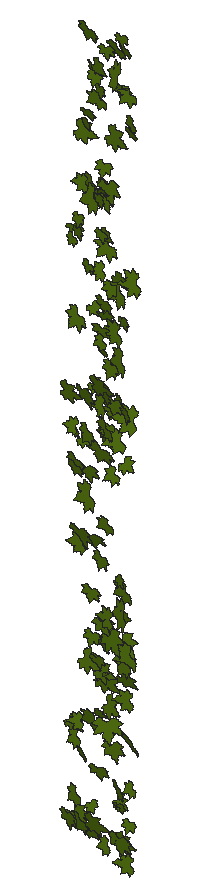
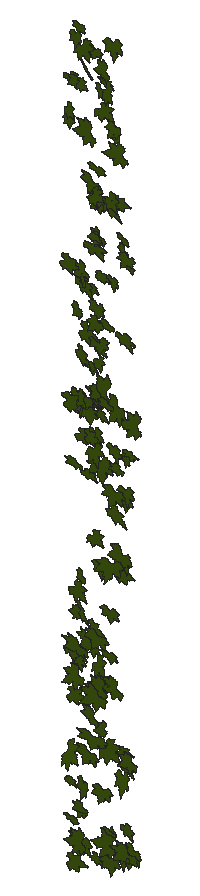
# SketchUp Ruby script. Lengths in inches.
U = 1.inch
M = Sketchup.active_model
def pt(a) = Geom::Point3d.new(a.map { |v| v * U })
def face(e, loops, mat)
  f = e.add_face(loops[0].map { |a| pt(a) })
  loops[1..].each { |l| e.add_face(l.map { |a| pt(a) }).erase! }
  f.material = f.back_material = mat if mat
  f
end
# faces: each face lists its corners as indices into pts; further lists are holes
def faces(e, pts, list, mat = nil) = list.each { |f| face(e, (f[0].is_a?(Array) ? f : [f]).map { |l| l.map { |i| pts[i] } }, mat) }
# xy, xz, yz: faces in a plane at the given z, y or x. An outline is a flat list of corners, or four numbers for a rectangle; further outlines are holes
def ring(l) = l.size == 4 ? [[l[0], l[1]], [l[2], l[1]], [l[2], l[3]], [l[0], l[3]]] : l.each_slice(2).to_a
def flat(e, list, mat, &to3) = list.each { |f| face(e, (f[0].is_a?(Array) ? f : [f]).map { |l| ring(l).map { |u, v| to3.(u, v) } }, mat) }
def xy(e, z, list, mat = nil) = flat(e, list, mat) { |x, y| [x, y, z] }
def xz(e, y, list, mat = nil) = flat(e, list, mat) { |x, z| [x, y, z] }
def yz(e, x, list, mat = nil) = flat(e, list, mat) { |y, z| [x, y, z] }
def lines(e, pts, list) = list.each { |a, b| e.add_line(pt(pts[a]), pt(pts[b])) }
# prism: a flat outline (further loops are holes) pulled along v
def prism(e, loops, v, mat = nil)
  f = face(e, loops, mat); d = Geom::Vector3d.new(v.map { |x| x * U })
  f.pushpull(f.normal.samedirection?(d) ? d.length : -d.length)
end
def box(e, o, s, mat = nil) = prism(e, [[o, [o[0] + s[0], o[1], o[2]], [o[0] + s[0], o[1] + s[1], o[2]], [o[0], o[1] + s[1], o[2]]]], [0, 0, s[2]], mat)
def at(x, y, z, deg = 0) = Geom::Transformation.translation(pt([x, y, z])) * Geom::Transformation.rotation(ORIGIN, Z_AXIS, deg.degrees)
def axes(o, x, y, z) = Geom::Transformation.new([*x, 0, *y, 0, *z, 0, *pt(o).to_a, 1])
def part(name) = M.definitions.add(name)
# library, detail: a bought-in or finely detailed component or shape, given as its bounding box
def library(name, o, s) = part(name).tap { |d| box(d.entities, o, s) }
def detail(e, o, s) = box(e.add_group.entities, o, s)
def put(e, d, t, mat = nil) = e.add_instance(d, t).tap { |i| i.material = mat if mat }
def group(e, t, mat = nil) = e.add_group.tap { |g| g.transformation = t; g.material = mat if mat }.entities
root = M.entities
M.materials.add("[Vegetation Blur 03]").color = [83, 114, 18]
c1 = part("ivy")
xy(c1.entities,0,[[0.782,0,0.786,0,0.787,0.005,0.789,0.009,0.821,0.072,0.875,0.147,1.001,0.272,1.073,0.331,1.137,0.363,1.178,0.379,1.223,0.384,1.272,0.383,1.311,0.374,1.36,0.355,1.399,0.334,1.491,0.285,1.541,0.244,1.583,0.199,1.617,0.15,1.64,0.128,1.662,0.115,1.717,0.105,1.745,0.093,1.784,0.054,1.819,0.057,1.854,0.064,1.882,0.075,1.896,0.074,1.91,0.071,1.937,0.063,1.964,0.053,1.99,0.038,2.016,0.015,2.034,0.002,2.04,0,2.038,0.003,2.036,0.007,2.033,0.038,2.036,0.068,2.045,0.1,2.055,0.116,2.064,0.123,2.077,0.129,2.088,0.129,2.106,0.132,2.118,0.13,2.179,0.132,2.207,0.133,2.225,0.133,2.242,0.138,2.22,0.162,2.207,0.186,2.206,0.213,2.212,0.236,2.228,0.262,2.247,0.274,2.298,0.283,2.355,0.294,2.37,0.296,2.376,0.295,2.377,0.3,2.377,0.303,2.385,0.329,2.411,0.37,2.426,0.392,2.449,0.407,2.511,0.426,2.561,0.444,2.619,0.466,2.589,0.469,2.561,0.476,2.501,0.5,2.449,0.516,2.424,0.523,2.401,0.535,2.377,0.556,2.372,0.568,2.36,0.575,2.268,0.586,2.225,0.592,2.207,0.599,2.194,0.61,2.143,0.65,2.13,0.664,2.122,0.682,2.123,0.7,2.13,0.719,2.148,0.75,2.17,0.781,2.195,0.807,2.221,0.828,2.284,0.874,2.291,0.88,2.288,0.887,2.276,0.9,2.267,0.916,2.265,0.933,2.273,0.967,2.292,1.002,2.313,1.03,2.334,1.054,2.348,1.067,2.358,1.074,2.363,1.076,2.362,1.081,2.35,1.094,2.347,1.11,2.35,1.143,2.359,1.18,2.385,1.254,2.415,1.324,2.448,1.393,2.45,1.4,2.446,1.398,2.44,1.394,2.427,1.383,2.402,1.36,2.376,1.339,2.345,1.324,2.305,1.309,2.282,1.303,2.273,1.306,2.245,1.294,2.212,1.287,2.187,1.291,2.163,1.301,2.142,1.316,2.134,1.327,2.124,1.325,2.09,1.292,2.053,1.259,2.014,1.234,1.973,1.215,1.954,1.21,1.931,1.208,1.909,1.212,1.893,1.22,1.879,1.233,1.872,1.248,1.867,1.281,1.864,1.319,1.821,1.258,1.773,1.197,1.726,1.141,1.698,1.121,1.679,1.116,1.666,1.117,1.647,1.122,1.632,1.129,1.62,1.141,1.617,1.154,1.617,1.219,1.621,1.254,1.623,1.268,1.623,1.281,1.618,1.314,1.606,1.346,1.603,1.375,1.607,1.403,1.603,1.467,1.599,1.499,1.605,1.525,1.614,1.552,1.629,1.577,1.635,1.589,1.629,1.587,1.618,1.582,1.596,1.566,1.581,1.556,1.568,1.552,1.557,1.55,1.545,1.553,1.531,1.562,1.522,1.572,1.504,1.591,1.486,1.611,1.474,1.631,1.457,1.666,1.455,1.684,1.457,1.698,1.452,1.715,1.444,1.728,1.424,1.754,1.419,1.772,1.423,1.786,1.434,1.819,1.444,1.848,1.446,1.855,1.44,1.861,1.43,1.867,1.386,1.904,1.349,1.948,1.326,1.973,1.31,1.995,1.288,2.048,1.284,2.153,1.287,2.254,1.284,2.255,1.282,2.253,1.278,2.247,1.274,2.237,1.266,2.216,1.226,2.125,1.208,2.076,1.184,2.033,1.155,1.984,1.135,1.942,1.111,1.899,1.083,1.861,1.053,1.85,1.059,1.83,1.061,1.809,1.056,1.79,1.049,1.767,1.04,1.749,1.018,1.733,0.994,1.726,0.942,1.734,0.95,1.6875,0.944,1.645,0.932,1.608,0.911,1.585,0.881,1.58,0.854,1.582,0.828,1.588,0.785,1.618,0.773,1.625,0.775,1.614,0.779,1.598,0.796,1.502,0.818,1.402,0.861,1.283,0.882,1.224,0.894,1.174,0.892,1.148,0.886,1.123,0.881,1.107,0.872,1.099,0.849,1.094,0.818,1.092,0.789,1.098,0.762,1.107,0.753,1.113,0.721,1.139,0.698,1.163,0.678,1.194,0.665,1.224,0.628,1.28,0.612,1.312,0.606,1.327,0.606,1.314,0.599,1.282,0.594,1.267,0.581,1.256,0.544,1.245,0.512,1.244,0.473,1.249,0.444,1.256,0.382,1.288,0.339,1.306,0.324,1.316,0.317,1.324,0.309,1.326,0.27,1.314,0.227,1.313,0.185,1.3125,0.152,1.317,0.122,1.328,0.092,1.345,0.073,1.353,0.079,1.338,0.092,1.308,0.117,1.249,0.13,1.215,0.139,1.164,0.147,1.148,0.157,1.136,0.163,1.122,0.174,1.086,0.177,1.067,0.182,1.054,0.186,1.043,0.191,1.038,0.211,1.028,0.237,1.005,0.25,0.974,0.253,0.96,0.25,0.944,0.242,0.914,0.243,0.906,0.249,0.902,0.26,0.894,0.289,0.88,0.307,0.873,0.322,0.862,0.364,0.799,0.403,0.738,0.431,0.709,0.439,0.691,0.441,0.678,0.4375,0.66,0.428,0.645,0.394,0.623,0.303,0.594,0.255,0.581,0.214,0.577,0.179,0.573,0.173,0.568,0.175,0.561,0.167,0.55,0.141,0.523,0.113,0.503,0.077,0.49,0.045,0.486,0.026,0.485,0.019,0.486,0.011,0.483,0,0.471,0.014,0.467,0.044,0.455,0.058,0.447,0.07,0.438,0.097,0.411,0.125,0.394,0.158,0.377,0.174,0.366,0.182,0.359,0.185,0.361,0.242,0.331,0.253,0.316,0.258,0.303,0.262,0.283,0.274,0.278,0.308,0.274,0.341,0.252,0.366,0.226,0.366,0.222,0.37,0.22,0.38,0.221,0.395,0.221,0.425,0.216,0.45,0.207,0.465,0.192,0.473,0.178,0.484,0.15,0.489,0.116,0.483,0.089,0.468,0.058,0.45,0.035,0.435,0.018,0.429,0.011,0.434,0.012,0.438,0.014,0.469,0.019,0.542,0.016,0.581,0.015,0.612,0.027,0.68,0.055,0.696,0.057,0.712,0.052,0.73,0.045,0.741,0.036,0.766,0.014]])
put(root,c1,axes([118.79,173.7,103.93],[0.51714,-0.23527,0.06533],[0.0842,0.02179,-0.43163],[-0.1113,-1.07662,-0.02301]),"[Vegetation Blur 03]")
put(root,c1,axes([119.9,173.7,124.375],[0.04403,-0.12753,-0.27738],[-0.34532,-0.03734,-0.03381],[0.01033,-0.70424,0.05202]),"[Vegetation Blur 03]")
put(root,c1,axes([119.375,173.7,133.94],[0.27643,-0.11245,-0.0959],[-0.1208,-0.01738,-0.22873],[-0.04691,-0.61786,0.02389]),"[Vegetation Blur 03]")
put(root,c1,axes([118.87,173.7,125.11],[0.08822,-0.12322,0.46198],[0.56917,0.00464,-0.0722],[-0.00698,-1.17889,-0.04857]),"[Vegetation Blur 03]")
put(root,c1,axes([119.09,173.7,134.17],[0.33638,0.01493,0.11781],[0.14294,0.07701,-0.27338],[0.02139,-0.74929,-0.02575]),"[Vegetation Blur 03]")
put(root,c1,axes([119.55,173.7,105.4],[0.34978,-0.17504,-0.23097],[-0.28247,0.06704,-0.29293],[-0.08681,-0.92345,0.02252]),"[Vegetation Blur 03]")
put(root,c1,axes([118.95,173.7,108.24],[0.25126,-0.00237,0.3092],[0.37875,0.02524,-0.20497],[0.00958,-0.93516,-0.00632]),"[Vegetation Blur 03]")
put(root,c1,axes([119.3,173.7,122.54],[0.44154,-0.10792,-0.13293],[-0.15664,0.11844,-0.36167],[-0.06888,-0.96117,-0.02964]),"[Vegetation Blur 03]")
put(root,c1,axes([119.32,173.7,122.13],[0.39751,-0.09835,-0.09675],[-0.112,0.11608,-0.32505],[-0.0616,-0.84567,-0.03337]),"[Vegetation Blur 03]")
put(root,c1,axes([120.2,173.7,118.44],[0.06394,-0.03491,-0.38067],[-0.46672,-0.01334,-0.05203],[0.00412,-0.96871,0.01444]),"[Vegetation Blur 03]")
put(root,c1,axes([119.71,173.7,108.375],[0.28202,-0.18926,-0.22565],[-0.28437,-0.00619,-0.23592],[-0.06351,-0.81269,0.05435]),"[Vegetation Blur 03]")
put(root,c1,axes([119.47,173.7,123.98],[0.28723,-0.15203,-0.02555],[-0.02588,0.0511,-0.24162],[-0.07595,-0.59236,-0.01429]),"[Vegetation Blur 03]")
put(root,c1,axes([120.08,173.7,109.22],[0.11929,-0.10597,-0.2818],[-0.34889,-0.06251,-0.09467],[0.01224,-0.74914,0.04776]),"[Vegetation Blur 03]")
put(root,c1,axes([119.54,173.7,130.3],[0.50454,-0.20666,-0.19788],[-0.2502,-0.0525,-0.4163],[-0.0792,-1.15072,0.05453]),"[Vegetation Blur 03]")
put(root,c1,axes([118.85,173.7,103.51],[0.43162,0.02667,0.37239],[0.45622,0.01814,-0.35241],[0.01531,-1.29236,0.00274]),"[Vegetation Blur 03]")
put(root,c1,axes([119.5,173.7,107.9],[0.51252,-0.27009,-0.18144],[-0.18784,0.30748,-0.42542],[-0.17711,-1.10772,-0.07385]),"[Vegetation Blur 03]")
put(root,c1,axes([119.56,173.7,104.04],[0.4822,-0.17189,-0.16775],[-0.19534,0.15084,-0.39833],[-0.10519,-1.06807,-0.02926]),"[Vegetation Blur 03]")
put(root,c1,axes([120.39,173.7,137.16],[0.05825,-0.05857,-0.32384],[-0.39732,-0.0501,-0.04618],[0.02002,-0.82377,0.02584]),"[Vegetation Blur 03]")
put(root,c1,axes([119.58,173.7,135.01],[0.33002,-0.10362,0.05882],[0.06392,-0.11285,-0.27012],[-0.06037,-0.68589,0.03556]),"[Vegetation Blur 03]")
put(root,c1,axes([119.53,173.7,134.21],[0.29872,-0.15455,0.15212],[0.18312,-0.07365,-0.25129],[-0.08276,-0.72081,-0.00694]),"[Vegetation Blur 03]")
put(root,c1,axes([119.71,173.7,123.02],[0.11399,0.08931,0.26369],[0.32563,0.00233,-0.09389],[0.01551,-0.70503,0.03309]),"[Vegetation Blur 03]")
put(root,c1,axes([119.25,173.7,118.8],[0.63866,-0.23189,0.12864],[0.16822,0.10928,-0.52532],[-0.09614,-1.34925,-0.06466]),"[Vegetation Blur 03]")
put(root,c1,axes([120.54,173.7,109.51],[0.24902,0.09318,-0.40988],[-0.50306,0.12516,-0.1991],[-0.03467,-1.14673,-0.05504]),"[Vegetation Blur 03]")
put(root,c1,axes([119.55,173.7,138.76],[0.09049,0.02962,0.47011],[0.57571,0.04471,-0.07426],[0.0237,-1.19903,0.00884]),"[Vegetation Blur 03]")
put(root,c1,axes([120.66,173.7,142.97],[0.14161,0.02749,-0.37414],[-0.43235,0.33737,-0.1051],[-0.153,-0.92792,-0.0493]),"[Vegetation Blur 03]")
put(root,c1,axes([120.43,173.7,121.4375],[0.39569,-0.25539,-0.40505],[-0.50198,0.05522,-0.33211],[-0.09868,-1.305,0.06522]),"[Vegetation Blur 03]")
put(root,c1,axes([119.92,173.7,145.125],[0.51011,-0.11701,-0.13612],[-0.15838,0.15628,-0.41647],[-0.07724,-1.09327,-0.04497]),"[Vegetation Blur 03]")
put(root,c1,axes([120.43,173.7,137.34],[0.31562,-0.0779,-0.30416],[-0.3657,0.1532,-0.25894],[-0.08116,-0.99323,-0.01608]),"[Vegetation Blur 03]")
put(root,c1,axes([120.03,173.7,103.54],[0.43132,0.00683,-0.12215],[-0.14822,0.15148,-0.34728],[-0.02104,-0.9272,-0.05763]),"[Vegetation Blur 03]")
put(root,c1,axes([119.72,173.7,118.54],[0.54712,0.06533,0.00829],[0.00324,0.23778,-0.43729],[0.03318,-1.10066,-0.09398]),"[Vegetation Blur 03]")
put(root,c1,axes([119.68,173.7,122.03],[0.51598,-0.04836,0.08245],[0.10256,0.07999,-0.4201],[-0.01553,-1.07898,-0.03484]),"[Vegetation Blur 03]")
put(root,c1,axes([120.11,173.7,124.36],[0.44792,-0.20906,-0.13241],[-0.16237,0.03502,-0.37455],[-0.10139,-0.9797,0.01487]),"[Vegetation Blur 03]")
put(root,c1,axes([119.91,173.7,140.5],[0.35213,-0.1038,0.09821],[0.12718,0.11373,-0.28482],[-0.02917,-0.75727,-0.05624]),"[Vegetation Blur 03]")
put(root,c1,axes([120.21,173.7,132.87],[0.35103,-0.1488,-0.07514],[-0.0909,0.03087,-0.29249],[-0.07377,-0.74614,0.00288]),"[Vegetation Blur 03]")
put(root,c1,axes([120.04,173.7,139.92],[0.22551,-0.17157,0.19026],[0.23404,-0.06401,-0.19384],[-0.08079,-0.66437,-0.03046]),"[Vegetation Blur 03]")
put(root,c1,axes([120.7,173.7,136.93],[0.36429,-0.26691,-0.39719],[-0.49048,0.09297,-0.30946],[-0.1145,-1.24751,0.06192]),"[Vegetation Blur 03]")
put(root,c1,axes([119.75,173.7,111.54],[0.19537,0.05525,0.44525],[0.54604,-0.05051,-0.1586],[-0.01409,-1.19141,0.02737]),"[Vegetation Blur 03]")
put(root,c1,axes([119.64,173.7,126.11],[0.57292,-0.29787,0.17247],[0.22282,0.05394,-0.47834],[-0.12636,-1.25544,-0.06147]),"[Vegetation Blur 03]")
put(root,c1,axes([120.13,173.7,115.97],[0.45876,-0.06676,-0.02085],[-0.02631,-0.02088,-0.37522],[-0.03182,-0.94526,0.00976]),"[Vegetation Blur 03]")
put(root,c1,axes([120.23,173.7,104.47],[0.21181,0.06558,0.16158],[0.19963,-0.12494,-0.16633],[-0.01894,-0.58339,0.05378]),"[Vegetation Blur 03]")
put(root,c1,axes([120.875,173.7,141.78],[0.26725,0.04128,-0.32232],[-0.39537,0.00799,-0.21819],[0.00802,-0.98126,-0.01534]),"[Vegetation Blur 03]")
put(root,c1,axes([120.28,173.7,113.7],[0.40879,-0.06868,-0.00639],[-0.01176,-0.09983,-0.33231],[-0.0322,-0.83542,0.04024]),"[Vegetation Blur 03]")
put(root,c1,axes([120.27,173.7,130.23],[0.21448,0.07418,0.20841],[0.25788,-0.06923,-0.1729],[-0.00284,-0.68276,0.04017]),"[Vegetation Blur 03]")
put(root,c1,axes([121.09,173.7,113.58],[0.21131,0.04206,-0.34485],[-0.41038,0.25638,-0.16258],[-0.10272,-0.93777,-0.05992]),"[Vegetation Blur 03]")
put(root,c1,axes([120.33,173.7,126.15],[0.18344,0.08958,0.24161],[0.29922,-0.05038,-0.14838],[0.0019,-0.7149,0.04073]),"[Vegetation Blur 03]")
put(root,c1,axes([120.5,173.7,142.72],[0.38042,-0.08348,0.02066],[0.01844,-0.12918,-0.30833],[-0.04412,-0.77385,0.04924]),"[Vegetation Blur 03]")
put(root,c1,axes([120.41,173.7,106.68],[0.44484,-0.01751,0.04002],[0.04967,0.10203,-0.36079],[-0.00297,-0.91526,-0.04099]),"[Vegetation Blur 03]")
put(root,c1,axes([120.47,173.7,112.36],[0.36338,-0.06137,0.0857],[0.10665,0.03955,-0.29676],[-0.02326,-0.77736,-0.02186]),"[Vegetation Blur 03]")
put(root,c1,axes([120.52,173.7,123.66],[0.62172,-0.07982,-0.18766],[-0.22411,0.16779,-0.50577],[-0.06444,-1.35373,-0.05162]),"[Vegetation Blur 03]")
put(root,c1,axes([121.01,173.7,128.71],[0.25042,-0.03463,-0.18206],[-0.21423,0.16131,-0.2011],[-0.06442,-0.671,-0.03895]),"[Vegetation Blur 03]")
put(root,c1,axes([121.46,173.7,137.26],[0.07231,0.11382,-0.30015],[-0.37128,0.06711,-0.05557],[-0.02172,-0.76837,-0.04931]),"[Vegetation Blur 03]")
put(root,c1,axes([121.36,173.7,133.02],[0.14335,-0.13764,-0.29117],[-0.36286,-0.03379,-0.11648],[-0.00945,-0.79049,0.05568]),"[Vegetation Blur 03]")
put(root,c1,axes([121.33,173.7,126.09],[0.18991,-0.19032,-0.31472],[-0.38839,0.08836,-0.16451],[-0.08006,-0.88012,0.05154]),"[Vegetation Blur 03]")
put(root,c1,axes([120.33,173.7,103.26],[0.11966,-0.19885,0.48664],[0.60405,0.04067,-0.09632],[0.00062,-1.25082,-0.0805]),"[Vegetation Blur 03]")
put(root,c1,axes([120.69,173.7,129.65],[0.43667,-0.00599,-0.05285],[-0.0643,0.07555,-0.35518],[-0.00825,-0.90526,-0.02929]),"[Vegetation Blur 03]")
put(root,c1,axes([121.19,173.7,129.25],[0.22039,-0.10268,-0.20891],[-0.2592,-0.01,-0.18136],[-0.02883,-0.69502,0.03347]),"[Vegetation Blur 03]")
put(root,c1,axes([121.1,173.7,124.3],[0.37381,-0.01776,-0.27785],[-0.3272,0.26974,-0.29592],[-0.09444,-1.00486,-0.07453]),"[Vegetation Blur 03]")
put(root,c1,axes([120.79,173.7,109.36],[0.12453,-0.12682,0.21988],[0.27637,0.0612,-0.0987],[0.00185,-0.60769,-0.05583]),"[Vegetation Blur 03]")
put(root,c1,axes([121.36,173.7,119.83],[0.24891,0.01709,-0.28911],[-0.35411,0.04401,-0.20266],[-0.01273,-0.88984,-0.01558]),"[Vegetation Blur 03]")
put(root,c1,axes([120.63,173.7,142.71],[0.15082,-0.08194,0.36497],[0.44384,-0.11913,-0.12637],[-0.06768,-0.96384,-0.01541]),"[Vegetation Blur 03]")
put(root,c1,axes([120.81,173.7,117.99],[0.46442,-0.17928,-0.04706],[-0.05947,-0.00913,-0.38545],[-0.0859,-0.96299,0.01241]),"[Vegetation Blur 03]")
put(root,c1,axes([120.76,173.7,136.34],[0.3125,-0.15896,0.12959],[0.15654,-0.05797,-0.26261],[-0.08171,-0.71898,-0.00748]),"[Vegetation Blur 03]")
put(root,c1,axes([121.8125,173.7,115.13],[0.07751,-0.08641,-0.39879],[-0.48715,0.10409,-0.06661],[-0.05668,-1.01274,0.02718]),"[Vegetation Blur 03]")
put(root,c1,axes([120.84,173.7,142.1],[0.3345,-0.16348,0.07359],[0.08724,-0.0471,-0.28058],[-0.08265,-0.71135,0.00167]),"[Vegetation Blur 03]")
put(root,c1,axes([120.8125,173.7,134.55],[0.32611,-0.0735,0.11387],[0.13621,-0.07341,-0.2673],[-0.04678,-0.72621,0.01549]),"[Vegetation Blur 03]")
put(root,c1,axes([121.52,173.7,103.31],[0.2031,-0.14404,-0.26055],[-0.32267,0.0347,-0.17055],[-0.052,-0.77785,0.04064]),"[Vegetation Blur 03]")
put(root,c1,axes([121.16,173.7,124.97],[0.45681,-0.21004,-0.23078],[-0.27305,0.15298,-0.3819],[-0.12578,-1.09491,-0.00909]),"[Vegetation Blur 03]")
put(root,c1,axes([120.73,173.7,111.1875],[0.0827,0.01826,0.45445],[0.55686,-0.01784,-0.06738],[-0.00727,-1.15829,0.0082]),"[Vegetation Blur 03]")
put(root,c1,axes([120.61,173.7,114.28],[0.50405,-0.0121,0.1413],[0.17315,0.00073,-0.4114],[-0.00545,-1.09673,-0.00183]),"[Vegetation Blur 03]")
put(root,c1,axes([120.82,173.7,136.54],[0.28631,-0.17737,0.19402],[0.25002,0.08801,-0.2331],[-0.03783,-0.76071,-0.07221]),"[Vegetation Blur 03]")
put(root,c1,axes([120.91,173.7,131.22],[0.46399,-0.15608,-0.0301],[-0.03246,0.06122,-0.3832],[-0.07784,-0.95586,-0.01963]),"[Vegetation Blur 03]")
put(root,c1,axes([120.85,173.7,130.17],[0.30561,-0.04373,0.17256],[0.21196,0.11676,-0.24539],[0.01507,-0.75575,-0.0479]),"[Vegetation Blur 03]")
put(root,c1,axes([120.96,173.7,138.21],[0.40348,-0.0468,0.02113],[0.02171,-0.14086,-0.32526],[-0.02676,-0.81998,0.05467]),"[Vegetation Blur 03]")
put(root,c1,axes([121.25,173.7,134.51],[0.49046,-0.12487,-0.25125],[-0.31171,-0.05916,-0.40067],[-0.03597,-1.19015,0.04628]),"[Vegetation Blur 03]")
put(root,c1,axes([120.75,173.7,126.02],[0.0827,-0.23642,0.52033],[0.64705,-0.03418,-0.07095],[-0.03151,-1.3225,-0.09118]),"[Vegetation Blur 03]")
put(root,c1,axes([121.01,173.7,144.17],[0.38022,-0.03036,0.06928],[0.08439,-0.02832,-0.31043],[-0.01739,-0.80118,0.00835]),"[Vegetation Blur 03]")
put(root,c1,axes([122.03,173.7,124.72],[0.06632,-0.08264,-0.34848],[-0.42857,0.02082,-0.0551],[-0.0162,-0.88896,0.0311]),"[Vegetation Blur 03]")
put(root,c1,axes([121.02,173.7,126.4],[0.3929,-0.21833,0.06927],[0.09371,0.04854,-0.33],[-0.09838,-0.82573,-0.03771]),"[Vegetation Blur 03]")
put(root,c1,axes([120.63,173.7,110.95],[0.37722,-0.01424,0.37521],[0.45787,0.12358,-0.30587],[0.04206,-1.2175,-0.03543]),"[Vegetation Blur 03]")
put(root,c1,axes([120.88,173.7,136.21],[0.36838,-0.06003,0.20905],[0.25298,-0.09287,-0.30112],[-0.04965,-0.91861,0.01678]),"[Vegetation Blur 03]")
put(root,c1,axes([121.1,173.7,126.58],[0.28308,-0.16005,0.12566],[0.16212,0.03888,-0.23548],[-0.05892,-0.66197,-0.04421]),"[Vegetation Blur 03]")
put(root,c1,axes([121.03,173.7,134.23],[0.16779,-0.0883,0.30239],[0.37001,-0.06611,-0.13979],[-0.04708,-0.83437,-0.02093]),"[Vegetation Blur 03]")
put(root,c1,axes([120.66,173.7,109.12],[0.61342,0.08443,0.16311],[0.20359,-0.16924,-0.49623],[0.01316,-1.31678,0.07424]),"[Vegetation Blur 03]")
put(root,c1,axes([122.18,173.7,130.22],[0.15478,-0.07462,-0.45486],[-0.55676,0.07347,-0.12809],[-0.04416,-1.18802,0.02065]),"[Vegetation Blur 03]")
put(root,c1,axes([121.79,173.7,144.67],[0.32569,0.04627,-0.29452],[-0.35796,0.18221,-0.25916],[-0.05099,-0.98359,-0.06186]),"[Vegetation Blur 03]")
put(root,c1,axes([121.44,173.7,125.87],[0.44969,-0.01244,-0.10758],[-0.13185,-0.00591,-0.36702],[-0.00499,-0.96429,0.00364]),"[Vegetation Blur 03]")
put(root,c1,axes([122.39,173.7,143.54],[0.07293,-0.28065,-0.423],[-0.50755,0.30955,-0.09059],[-0.17213,-1.03162,0.0879]),"[Vegetation Blur 03]")
put(root,c1,axes([121.38,173.7,132.12],[0.43256,-0.06671,-0.01604],[-0.02325,-0.10108,-0.35159],[-0.02994,-0.88528,0.04135]),"[Vegetation Blur 03]")
put(root,c1,axes([121.875,173.7,122.7],[0.28967,-0.12811,-0.2275],[-0.2852,-0.08534,-0.23432],[-0.01552,-0.82284,0.05972]),"[Vegetation Blur 03]")
put(root,c1,axes([121.18,173.7,109.63],[0.13579,0.06981,0.42324],[0.51409,-0.17958,-0.1052],[-0.07611,-1.08841,0.0445]),"[Vegetation Blur 03]")
put(root,c1,axes([121.43,173.7,128.09],[0.442,-0.16404,-0.03453],[-0.05057,-0.08968,-0.36412],[-0.07475,-0.90929,0.04214]),"[Vegetation Blur 03]")
put(root,c1,axes([120.96,173.7,137.1],[0.56013,-0.13091,0.22183],[0.26451,-0.15182,-0.45897],[-0.08921,-1.27215,0.03195]),"[Vegetation Blur 03]")
put(root,c1,axes([121.18,173.7,108.09],[0.51003,-0.05161,0.17077],[0.20792,-0.06034,-0.4165],[-0.03431,-1.13281,0.01441]),"[Vegetation Blur 03]")
put(root,c1,axes([122.26,173.7,142.51],[0.10604,0.023,-0.23018],[-0.28135,0.05824,-0.08542],[-0.02259,-0.61729,-0.01663]),"[Vegetation Blur 03]")
put(root,c1,axes([122.27,173.7,124.7],[0.25465,-0.11048,-0.36792],[-0.45313,-0.12762,-0.20287],[0.02807,-1.05778,0.0629]),"[Vegetation Blur 03]")
put(root,c1,axes([121.06,173.7,113.4375],[0.45366,-0.05419,0.38117],[0.46073,-0.18,-0.36926],[-0.08098,-1.3277,0.0345]),"[Vegetation Blur 03]")
put(root,c1,axes([121.46,173.7,126.17],[0.49069,-0.15556,0.05335],[0.06086,-0.06942,-0.40473],[-0.07927,-1.0163,0.01948]),"[Vegetation Blur 03]")
put(root,c1,axes([122.36,173.7,128.93],[0.29092,-0.24551,-0.40873],[-0.49509,0.19114,-0.25278],[-0.14116,-1.1764,0.04423]),"[Vegetation Blur 03]")
put(root,c1,axes([122.1,173.7,132.52],[0.43677,-0.25618,-0.34823],[-0.42807,0.08886,-0.36791],[-0.11962,-1.25334,0.04509]),"[Vegetation Blur 03]")
put(root,c1,axes([122.52,173.7,115.91],[0.26701,-0.30376,-0.4486],[-0.53833,0.27065,-0.24226],[-0.1847,-1.22801,0.05757]),"[Vegetation Blur 03]")
put(root,c1,axes([121.35,173.7,139.19],[0.18628,-0.03587,0.49266],[0.60208,-0.08964,-0.15266],[-0.04677,-1.29689,-0.00307]),"[Vegetation Blur 03]")
put(root,c1,axes([122.78,173.7,108.76],[0.09506,0.21771,-0.46057],[-0.55663,0.32363,-0.05246],[-0.14082,-1.13231,-0.10355]),"[Vegetation Blur 03]")
put(root,c1,axes([122.41,173.7,116.89],[0.30205,-0.06223,-0.36549],[-0.44449,0.11303,-0.2477],[-0.06243,-1.1058,-0.00475]),"[Vegetation Blur 03]")
put(root,c1,axes([121.84,173.7,105.14],[0.28399,-0.06546,0.07539],[0.09562,0.06624,-0.23087],[-0.02006,-0.61097,-0.03311]),"[Vegetation Blur 03]")
put(root,c1,axes([121.77,173.7,105.02],[0.18546,0.05213,0.26962],[0.33131,-0.03649,-0.15069],[-0.00311,-0.77875,0.02511]),"[Vegetation Blur 03]")
put(root,c1,axes([121.85,173.7,106.47],[0.46353,-0.32199,-0.04056],[-0.03174,0.12476,-0.39742],[-0.16108,-0.95117,-0.0384]),"[Vegetation Blur 03]")
put(root,c1,axes([121.72,173.7,132.26],[0.26264,-0.10696,0.28896],[0.35555,-0.0243,-0.21667],[-0.0405,-0.90682,-0.02828]),"[Vegetation Blur 03]")
put(root,c1,axes([121.58,173.7,103.66],[0.62439,-0.15847,0.04406],[0.05688,0.04229,-0.51297],[-0.0749,-1.28898,-0.02225]),"[Vegetation Blur 03]")
put(root,c1,axes([122,173.7,145.09],[0.3174,-0.05029,0.04385],[0.05287,-0.02687,-0.25971],[-0.02626,-0.66189,0.00721]),"[Vegetation Blur 03]")
put(root,c1,axes([121.97,173.7,116.77],[0.18692,-0.08145,0.20202],[0.24238,-0.1034,-0.15594],[-0.06396,-0.62987,-0.00053]),"[Vegetation Blur 03]")
put(root,c1,axes([122.09,173.7,126.54],[0.55558,-0.31709,-0.23093],[-0.26347,0.22092,-0.46992],[-0.18545,-1.26384,-0.0242]),"[Vegetation Blur 03]")
put(root,c1,axes([122.9375,173.7,111.32],[0.10909,-0.05884,-0.38294],[-0.46937,-0.06819,-0.08742],[0.02587,-0.98895,0.02881]),"[Vegetation Blur 03]")
put(root,c1,axes([123.01,173.7,102.81],[0.07011,-0.04175,-0.39035],[-0.47768,-0.07166,-0.05594],[0.03155,-0.99215,0.02047]),"[Vegetation Blur 03]")
put(root,c1,axes([122.23,173.7,144.76],[0.35771,-0.12648,-0.10441],[-0.11497,0.1604,-0.29291],[-0.08323,-0.76513,-0.04414]),"[Vegetation Blur 03]")
put(root,c1,axes([122.19,173.7,113.06],[0.4568,-0.18649,-0.14633],[-0.18134,0.01163,-0.3794],[-0.08646,-1.00976,0.02265]),"[Vegetation Blur 03]")
put(root,c1,axes([122.73,173.7,113.83],[0.34831,-0.13161,-0.42418],[-0.52189,0.01831,-0.28634],[-0.04303,-1.28736,0.03929]),"[Vegetation Blur 03]")
put(root,c1,axes([122.09,173.7,122.53],[0.15249,0.14355,0.27563],[0.34484,-0.05498,-0.12257],[0.00385,-0.76056,0.06089]),"[Vegetation Blur 03]")
put(root,c1,axes([121.67,173.7,113.11],[0.33086,0.13392,0.42114],[0.51995,-0.11554,-0.26631],[-0.01255,-1.25609,0.0694]),"[Vegetation Blur 03]")
put(root,c1,axes([122.1875,173.7,142.08],[0.20167,-0.04503,0.17751],[0.21848,0.0617,-0.16287],[0.00725,-0.60725,-0.02971]),"[Vegetation Blur 03]")
put(root,c1,axes([122.33,173.7,114.78],[0.04043,-0.04833,0.23762],[0.29161,-0.02839,-0.03396],[-0.01694,-0.60422,-0.01741]),"[Vegetation Blur 03]")
put(root,c1,axes([122.14,173.7,130.4],[0.29752,-0.1463,0.14185],[0.17418,-0.03541,-0.24908],[-0.07018,-0.70816,-0.01685]),"[Vegetation Blur 03]")
put(root,c1,axes([121.99,173.7,102.9],[0.12855,-0.09811,0.43066],[0.52964,-0.00555,-0.1055],[-0.01392,-1.1176,-0.03728]),"[Vegetation Blur 03]")
put(root,c1,axes([122.92,173.7,141.07],[0.17412,-0.05091,-0.27988],[-0.33267,0.17495,-0.14285],[-0.08689,-0.77186,-0.01392]),"[Vegetation Blur 03]")
put(root,c1,axes([123.375,173.7,126.18],[0.08303,-0.1967,-0.5076],[-0.62878,-0.07669,-0.06383],[0.02474,-1.28895,0.08126]),"[Vegetation Blur 03]")
put(root,c1,axes([122.59,173.7,142.65],[0.37323,-0.08724,-0.21133],[-0.2619,-0.06711,-0.30372],[-0.01607,-0.93236,0.04164]),"[Vegetation Blur 03]")
put(root,c1,axes([121.96,173.7,111.6],[0.33482,-0.12296,0.29954],[0.37174,0.13576,-0.26801],[0.00918,-1.01326,-0.07226]),"[Vegetation Blur 03]")
put(root,c1,axes([122.625,173.7,140.47],[0.29211,-0.05666,-0.12031],[-0.1385,0.15286,-0.23529],[-0.05752,-0.65573,-0.04445]),"[Vegetation Blur 03]")
put(root,c1,axes([122.9375,173.7,106.68],[0.22279,-0.12525,-0.19809],[-0.24846,-0.03124,-0.18302],[-0.02974,-0.67725,0.04508]),"[Vegetation Blur 03]")
put(root,c1,axes([122.52,173.7,104.61],[0.33968,-0.06301,-0.00772],[-0.01455,-0.11855,-0.2742],[-0.02856,-0.68915,0.04788]),"[Vegetation Blur 03]")
put(root,c1,axes([123.28,173.7,133.27],[0.22309,-0.1604,-0.43567],[-0.53899,-0.01598,-0.18291],[-0.02282,-1.19045,0.06116]),"[Vegetation Blur 03]")
